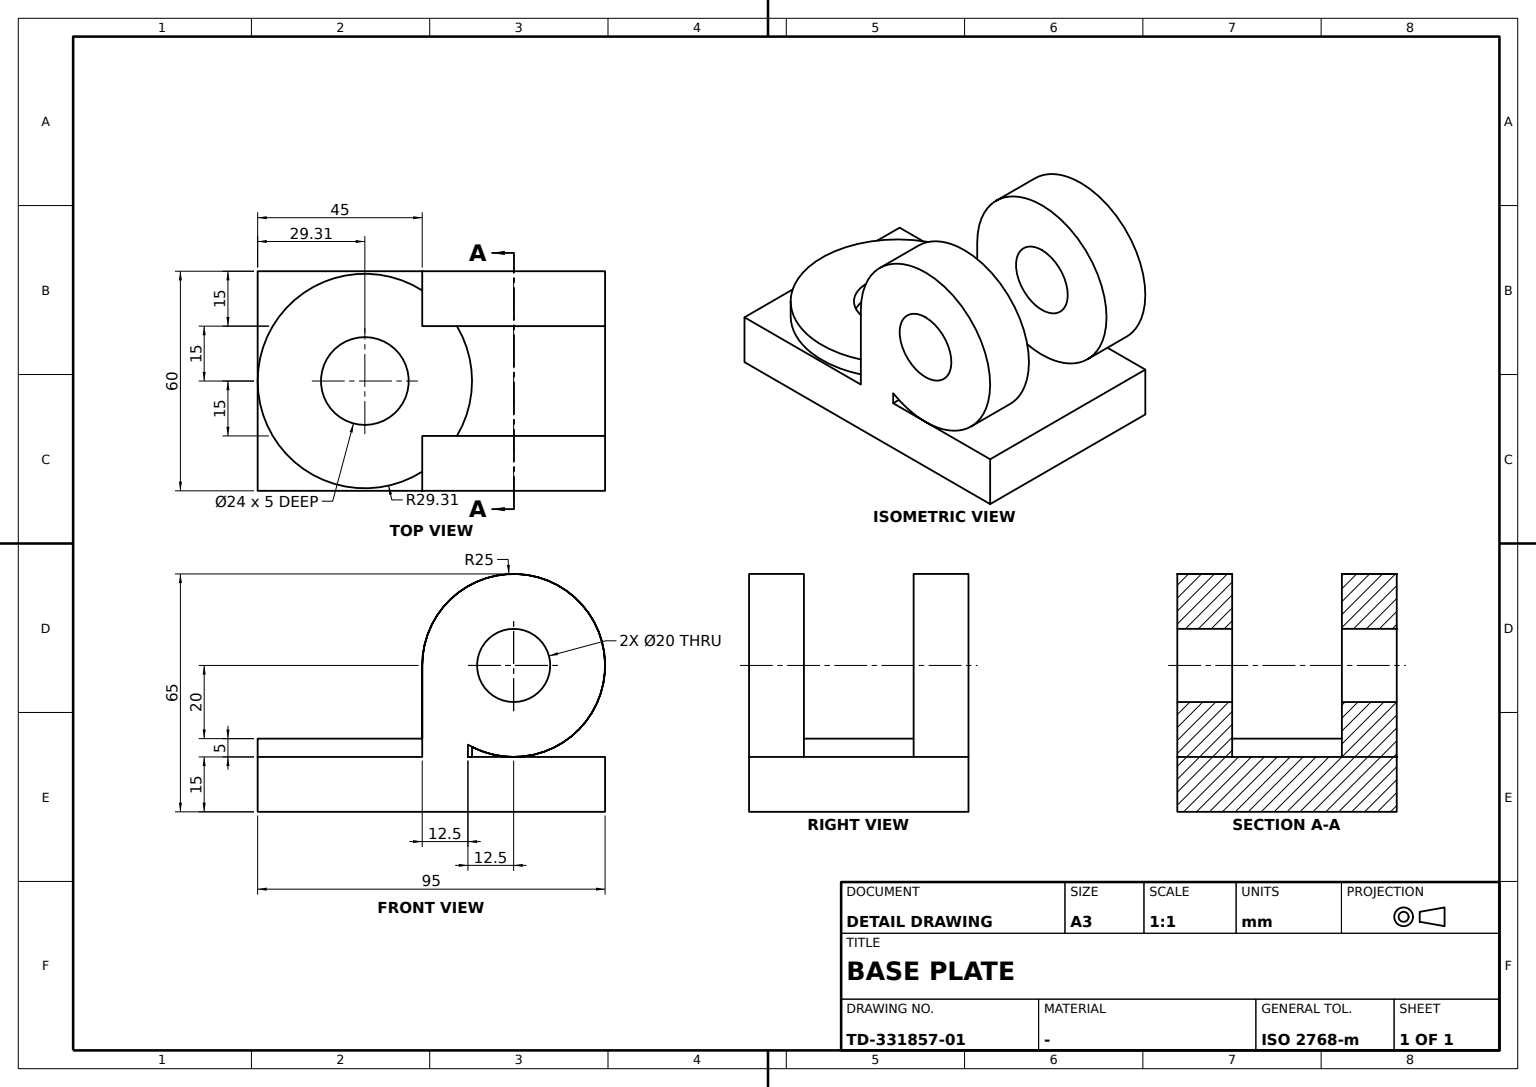
ISO-10303-21;
HEADER;
FILE_DESCRIPTION((''),'2;1');
FILE_NAME('','',(''),(''),'','','');
FILE_SCHEMA(('AUTOMOTIVE_DESIGN'));
ENDSEC;
DATA;
#1=APPLICATION_CONTEXT('');
#2=PRODUCT_CONTEXT('',#1,'mechanical');
#3=PRODUCT('','','',(#2));
#4=PRODUCT_DEFINITION_FORMATION('','',#3);
#5=PRODUCT_DEFINITION_CONTEXT('',#1,'design');
#6=PRODUCT_DEFINITION('','',#4,#5);
#7=PRODUCT_DEFINITION_SHAPE('','',#6);
#8=(LENGTH_UNIT()NAMED_UNIT(*)SI_UNIT(.MILLI.,.METRE.));
#9=(NAMED_UNIT(*)PLANE_ANGLE_UNIT()SI_UNIT($,.RADIAN.));
#10=(NAMED_UNIT(*)SI_UNIT($,.STERADIAN.)SOLID_ANGLE_UNIT());
#11=UNCERTAINTY_MEASURE_WITH_UNIT(LENGTH_MEASURE(0.005),#8,'distance_accuracy_value','');
#12=(GEOMETRIC_REPRESENTATION_CONTEXT(3)GLOBAL_UNCERTAINTY_ASSIGNED_CONTEXT((#11))GLOBAL_UNIT_ASSIGNED_CONTEXT((#8,#9,#10))REPRESENTATION_CONTEXT('',''));
#13=CARTESIAN_POINT('',(-15.,22.5,50.));
#14=VERTEX_POINT('',#13);
#15=CARTESIAN_POINT('',(-15.,22.5,40.));
#16=DIRECTION('',(-1.,0.,0.));
#17=DIRECTION('',(0.,0.,1.));
#18=AXIS2_PLACEMENT_3D('',#15,#16,#17);
#19=CIRCLE('',#18,10.);
#20=EDGE_CURVE('',#14,#14,#19,.T.);
#21=ORIENTED_EDGE('',*,*,#20,.T.);
#22=EDGE_LOOP('',(#21));
#23=FACE_BOUND('',#22,.T.);
#24=CARTESIAN_POINT('',(-15.,-2.5,40.));
#25=VERTEX_POINT('',#24);
#26=CARTESIAN_POINT('',(-15.,10.,18.349365));
#27=VERTEX_POINT('',#26);
#28=CIRCLE('',#18,25.);
#29=EDGE_CURVE('',#25,#27,#28,.T.);
#30=ORIENTED_EDGE('',*,*,#29,.F.);
#31=CARTESIAN_POINT('',(-15.,-2.5,20.));
#32=VERTEX_POINT('',#31);
#33=DIRECTION('',(0.,0.,-1.));
#34=VECTOR('',#33,1000.);
#35=LINE('',#24,#34);
#36=EDGE_CURVE('',#25,#32,#35,.T.);
#37=ORIENTED_EDGE('',*,*,#36,.T.);
#38=CARTESIAN_POINT('',(-15.,6.991539,20.));
#39=VERTEX_POINT('',#38);
#40=CARTESIAN_POINT('',(-15.,0.,20.));
#41=DIRECTION('',(0.,-1.,0.));
#42=VECTOR('',#41,1000.);
#43=LINE('',#40,#42);
#44=EDGE_CURVE('',#39,#32,#43,.T.);
#45=ORIENTED_EDGE('',*,*,#44,.F.);
#46=CARTESIAN_POINT('',(-15.,6.991539,15.));
#47=VERTEX_POINT('',#46);
#48=VECTOR('',#17,1000.);
#49=LINE('',#46,#48);
#50=EDGE_CURVE('',#47,#39,#49,.T.);
#51=ORIENTED_EDGE('',*,*,#50,.F.);
#52=CARTESIAN_POINT('',(-15.,10.,15.));
#53=VERTEX_POINT('',#52);
#54=CARTESIAN_POINT('',(-15.,0.,15.));
#55=DIRECTION('',(0.,1.,0.));
#56=VECTOR('',#55,1000.);
#57=LINE('',#54,#56);
#58=EDGE_CURVE('',#47,#53,#57,.T.);
#59=ORIENTED_EDGE('',*,*,#58,.T.);
#60=LINE('',#52,#48);
#61=EDGE_CURVE('',#53,#27,#60,.T.);
#62=ORIENTED_EDGE('',*,*,#61,.T.);
#63=EDGE_LOOP('',(#30,#37,#45,#51,#59,#62));
#64=FACE_BOUND('',#63,.T.);
#65=CARTESIAN_POINT('',(-15.,0.,0.));
#66=AXIS2_PLACEMENT_3D('',#65,#16,#41);
#67=PLANE('',#66);
#68=ADVANCED_FACE('',(#23,#64),#67,.F.);
#69=CARTESIAN_POINT('',(-24.757381,-2.5,20.));
#70=VERTEX_POINT('',#69);
#71=CARTESIAN_POINT('',(24.757381,-2.5,20.));
#72=VERTEX_POINT('',#71);
#73=CARTESIAN_POINT('',(0.,-18.18969,20.));
#74=DIRECTION('',(1.,0.,0.));
#75=AXIS2_PLACEMENT_3D('',#73,#17,#74);
#76=CIRCLE('',#75,29.31031);
#77=EDGE_CURVE('',#70,#72,#76,.T.);
#78=ORIENTED_EDGE('',*,*,#77,.F.);
#79=CARTESIAN_POINT('',(-24.757381,-2.5,15.));
#80=VERTEX_POINT('',#79);
#81=LINE('',#79,#48);
#82=EDGE_CURVE('',#80,#70,#81,.T.);
#83=ORIENTED_EDGE('',*,*,#82,.F.);
#84=CARTESIAN_POINT('',(0.,-47.5,15.));
#85=VERTEX_POINT('',#84);
#86=CARTESIAN_POINT('',(0.,-18.18969,15.));
#87=AXIS2_PLACEMENT_3D('',#86,#17,#74);
#88=CIRCLE('',#87,29.31031);
#89=EDGE_CURVE('',#80,#85,#88,.T.);
#90=ORIENTED_EDGE('',*,*,#89,.T.);
#91=CARTESIAN_POINT('',(24.757381,-2.5,15.));
#92=VERTEX_POINT('',#91);
#93=EDGE_CURVE('',#85,#92,#88,.T.);
#94=ORIENTED_EDGE('',*,*,#93,.T.);
#95=LINE('',#91,#48);
#96=EDGE_CURVE('',#92,#72,#95,.T.);
#97=ORIENTED_EDGE('',*,*,#96,.T.);
#98=EDGE_LOOP('',(#78,#83,#90,#94,#97));
#99=FACE_BOUND('',#98,.T.);
#100=CARTESIAN_POINT('',(0.,-18.18969,17.5));
#101=AXIS2_PLACEMENT_3D('',#100,#17,#74);
#102=CYLINDRICAL_SURFACE('',#101,29.31031);
#103=ADVANCED_FACE('',(#99),#102,.T.);
#104=CARTESIAN_POINT('',(-30.,-2.5,40.));
#105=VERTEX_POINT('',#104);
#106=CARTESIAN_POINT('',(-30.,10.,18.349365));
#107=VERTEX_POINT('',#106);
#108=CARTESIAN_POINT('',(-30.,22.5,40.));
#109=AXIS2_PLACEMENT_3D('',#108,#16,#17);
#110=CIRCLE('',#109,25.);
#111=EDGE_CURVE('',#105,#107,#110,.T.);
#112=ORIENTED_EDGE('',*,*,#111,.F.);
#113=CARTESIAN_POINT('',(-22.5,-2.5,40.));
#114=VECTOR('',#16,1000.);
#115=LINE('',#113,#114);
#116=EDGE_CURVE('',#105,#25,#115,.F.);
#117=ORIENTED_EDGE('',*,*,#116,.T.);
#118=ORIENTED_EDGE('',*,*,#29,.T.);
#119=LINE('',#106,#114);
#120=EDGE_CURVE('',#107,#27,#119,.F.);
#121=ORIENTED_EDGE('',*,*,#120,.F.);
#122=EDGE_LOOP('',(#112,#117,#118,#121));
#123=FACE_BOUND('',#122,.T.);
#124=CARTESIAN_POINT('',(-22.5,22.5,40.));
#125=AXIS2_PLACEMENT_3D('',#124,#16,#41);
#126=CYLINDRICAL_SURFACE('',#125,25.);
#127=ADVANCED_FACE('',(#123),#126,.T.);
#128=CARTESIAN_POINT('',(12.,-18.18969,20.));
#129=VERTEX_POINT('',#128);
#130=CIRCLE('',#75,12.);
#131=EDGE_CURVE('',#129,#129,#130,.T.);
#132=ORIENTED_EDGE('',*,*,#131,.T.);
#133=EDGE_LOOP('',(#132));
#134=FACE_BOUND('',#133,.T.);
#135=CARTESIAN_POINT('',(12.,-18.18969,15.));
#136=VERTEX_POINT('',#135);
#137=CIRCLE('',#87,12.);
#138=EDGE_CURVE('',#136,#136,#137,.T.);
#139=ORIENTED_EDGE('',*,*,#138,.F.);
#140=EDGE_LOOP('',(#139));
#141=FACE_BOUND('',#140,.T.);
#142=CYLINDRICAL_SURFACE('',#101,12.);
#143=ADVANCED_FACE('',(#134,#141),#142,.F.);
#144=CARTESIAN_POINT('',(30.,22.5,15.));
#145=VERTEX_POINT('',#144);
#146=CARTESIAN_POINT('',(30.,10.,18.349365));
#147=VERTEX_POINT('',#146);
#148=CARTESIAN_POINT('',(30.,22.5,40.));
#149=AXIS2_PLACEMENT_3D('',#148,#16,#17);
#150=CIRCLE('',#149,25.);
#151=EDGE_CURVE('',#145,#147,#150,.T.);
#152=ORIENTED_EDGE('',*,*,#151,.T.);
#153=CARTESIAN_POINT('',(15.,10.,18.349365));
#154=VERTEX_POINT('',#153);
#155=LINE('',#153,#114);
#156=EDGE_CURVE('',#154,#147,#155,.F.);
#157=ORIENTED_EDGE('',*,*,#156,.F.);
#158=CARTESIAN_POINT('',(15.,-2.5,40.));
#159=VERTEX_POINT('',#158);
#160=CARTESIAN_POINT('',(15.,22.5,40.));
#161=AXIS2_PLACEMENT_3D('',#160,#16,#17);
#162=CIRCLE('',#161,25.);
#163=EDGE_CURVE('',#159,#154,#162,.T.);
#164=ORIENTED_EDGE('',*,*,#163,.F.);
#165=CARTESIAN_POINT('',(30.,-2.5,40.));
#166=VERTEX_POINT('',#165);
#167=EDGE_CURVE('',#159,#166,#115,.F.);
#168=ORIENTED_EDGE('',*,*,#167,.T.);
#169=EDGE_CURVE('',#166,#145,#150,.T.);
#170=ORIENTED_EDGE('',*,*,#169,.T.);
#171=EDGE_LOOP('',(#152,#157,#164,#168,#170));
#172=FACE_BOUND('',#171,.T.);
#173=ADVANCED_FACE('',(#172),#126,.T.);
#174=ORIENTED_EDGE('',*,*,#50,.T.);
#175=CARTESIAN_POINT('',(15.,6.991539,20.));
#176=VERTEX_POINT('',#175);
#177=EDGE_CURVE('',#176,#39,#76,.T.);
#178=ORIENTED_EDGE('',*,*,#177,.F.);
#179=CARTESIAN_POINT('',(15.,6.991539,15.));
#180=VERTEX_POINT('',#179);
#181=LINE('',#179,#48);
#182=EDGE_CURVE('',#180,#176,#181,.T.);
#183=ORIENTED_EDGE('',*,*,#182,.F.);
#184=EDGE_CURVE('',#180,#47,#88,.T.);
#185=ORIENTED_EDGE('',*,*,#184,.T.);
#186=EDGE_LOOP('',(#174,#178,#183,#185));
#187=FACE_BOUND('',#186,.T.);
#188=ADVANCED_FACE('',(#187),#102,.T.);
#189=ORIENTED_EDGE('',*,*,#138,.T.);
#190=EDGE_LOOP('',(#189));
#191=FACE_BOUND('',#190,.T.);
#192=CARTESIAN_POINT('',(0.,0.,15.));
#193=AXIS2_PLACEMENT_3D('',#192,#17,#74);
#194=PLANE('',#193);
#195=ADVANCED_FACE('',(#191),#194,.T.);
#196=CARTESIAN_POINT('',(-30.,22.5,50.));
#197=VERTEX_POINT('',#196);
#198=CIRCLE('',#109,10.);
#199=EDGE_CURVE('',#197,#197,#198,.T.);
#200=ORIENTED_EDGE('',*,*,#199,.T.);
#201=EDGE_LOOP('',(#200));
#202=FACE_BOUND('',#201,.T.);
#203=ORIENTED_EDGE('',*,*,#20,.F.);
#204=EDGE_LOOP('',(#203));
#205=FACE_BOUND('',#204,.T.);
#206=CYLINDRICAL_SURFACE('',#125,10.);
#207=ADVANCED_FACE('',(#202,#205),#206,.F.);
#208=CARTESIAN_POINT('',(-30.,47.5,0.));
#209=VERTEX_POINT('',#208);
#210=CARTESIAN_POINT('',(30.,47.5,0.));
#211=VERTEX_POINT('',#210);
#212=CARTESIAN_POINT('',(0.,47.5,0.));
#213=VECTOR('',#74,1000.);
#214=LINE('',#212,#213);
#215=EDGE_CURVE('',#209,#211,#214,.T.);
#216=ORIENTED_EDGE('',*,*,#215,.F.);
#217=CARTESIAN_POINT('',(-30.,47.5,15.));
#218=VERTEX_POINT('',#217);
#219=LINE('',#208,#48);
#220=EDGE_CURVE('',#209,#218,#219,.T.);
#221=ORIENTED_EDGE('',*,*,#220,.T.);
#222=CARTESIAN_POINT('',(30.,47.5,15.));
#223=VERTEX_POINT('',#222);
#224=CARTESIAN_POINT('',(0.,47.5,15.));
#225=LINE('',#224,#213);
#226=EDGE_CURVE('',#218,#223,#225,.T.);
#227=ORIENTED_EDGE('',*,*,#226,.T.);
#228=LINE('',#210,#48);
#229=EDGE_CURVE('',#211,#223,#228,.T.);
#230=ORIENTED_EDGE('',*,*,#229,.F.);
#231=EDGE_LOOP('',(#216,#221,#227,#230));
#232=FACE_BOUND('',#231,.T.);
#233=AXIS2_PLACEMENT_3D('',#208,#41,#74);
#234=PLANE('',#233);
#235=ADVANCED_FACE('',(#232),#234,.F.);
#236=CARTESIAN_POINT('',(-30.,-2.5,15.));
#237=VERTEX_POINT('',#236);
#238=LINE('',#104,#34);
#239=EDGE_CURVE('',#105,#237,#238,.T.);
#240=ORIENTED_EDGE('',*,*,#239,.F.);
#241=ORIENTED_EDGE('',*,*,#111,.T.);
#242=CARTESIAN_POINT('',(-30.,10.,15.));
#243=VERTEX_POINT('',#242);
#244=LINE('',#242,#48);
#245=EDGE_CURVE('',#243,#107,#244,.T.);
#246=ORIENTED_EDGE('',*,*,#245,.F.);
#247=CARTESIAN_POINT('',(-30.,0.,15.));
#248=LINE('',#247,#42);
#249=EDGE_CURVE('',#218,#243,#248,.T.);
#250=ORIENTED_EDGE('',*,*,#249,.F.);
#251=ORIENTED_EDGE('',*,*,#220,.F.);
#252=CARTESIAN_POINT('',(-30.,-47.5,0.));
#253=VERTEX_POINT('',#252);
#254=CARTESIAN_POINT('',(-30.,0.,0.));
#255=LINE('',#254,#42);
#256=EDGE_CURVE('',#209,#253,#255,.T.);
#257=ORIENTED_EDGE('',*,*,#256,.T.);
#258=CARTESIAN_POINT('',(-30.,-47.5,15.));
#259=VERTEX_POINT('',#258);
#260=LINE('',#252,#48);
#261=EDGE_CURVE('',#253,#259,#260,.T.);
#262=ORIENTED_EDGE('',*,*,#261,.T.);
#263=EDGE_CURVE('',#237,#259,#248,.T.);
#264=ORIENTED_EDGE('',*,*,#263,.F.);
#265=EDGE_LOOP('',(#240,#241,#246,#250,#251,#257,#262,#264));
#266=FACE_BOUND('',#265,.T.);
#267=ORIENTED_EDGE('',*,*,#199,.F.);
#268=EDGE_LOOP('',(#267));
#269=FACE_BOUND('',#268,.T.);
#270=AXIS2_PLACEMENT_3D('',#208,#16,#41);
#271=PLANE('',#270);
#272=ADVANCED_FACE('',(#266,#269),#271,.T.);
#273=CARTESIAN_POINT('',(15.,-2.5,20.));
#274=VERTEX_POINT('',#273);
#275=CARTESIAN_POINT('',(0.,-2.5,20.));
#276=LINE('',#275,#213);
#277=EDGE_CURVE('',#274,#72,#276,.T.);
#278=ORIENTED_EDGE('',*,*,#277,.T.);
#279=ORIENTED_EDGE('',*,*,#96,.F.);
#280=CARTESIAN_POINT('',(30.,-2.5,15.));
#281=VERTEX_POINT('',#280);
#282=CARTESIAN_POINT('',(0.,-2.5,15.));
#283=LINE('',#282,#213);
#284=EDGE_CURVE('',#92,#281,#283,.T.);
#285=ORIENTED_EDGE('',*,*,#284,.T.);
#286=LINE('',#165,#34);
#287=EDGE_CURVE('',#166,#281,#286,.T.);
#288=ORIENTED_EDGE('',*,*,#287,.F.);
#289=ORIENTED_EDGE('',*,*,#167,.F.);
#290=LINE('',#158,#34);
#291=EDGE_CURVE('',#159,#274,#290,.T.);
#292=ORIENTED_EDGE('',*,*,#291,.T.);
#293=EDGE_LOOP('',(#278,#279,#285,#288,#289,#292));
#294=FACE_BOUND('',#293,.T.);
#295=AXIS2_PLACEMENT_3D('',#104,#41,#33);
#296=PLANE('',#295);
#297=ADVANCED_FACE('',(#294),#296,.T.);
#298=ORIENTED_EDGE('',*,*,#61,.F.);
#299=LINE('',#242,#213);
#300=EDGE_CURVE('',#243,#53,#299,.T.);
#301=ORIENTED_EDGE('',*,*,#300,.F.);
#302=ORIENTED_EDGE('',*,*,#245,.T.);
#303=ORIENTED_EDGE('',*,*,#120,.T.);
#304=EDGE_LOOP('',(#298,#301,#302,#303));
#305=FACE_BOUND('',#304,.T.);
#306=AXIS2_PLACEMENT_3D('',#242,#55,#17);
#307=PLANE('',#306);
#308=ADVANCED_FACE('',(#305),#307,.T.);
#309=ORIENTED_EDGE('',*,*,#215,.T.);
#310=CARTESIAN_POINT('',(30.,-47.5,0.));
#311=VERTEX_POINT('',#310);
#312=LINE('',#210,#56);
#313=EDGE_CURVE('',#311,#211,#312,.T.);
#314=ORIENTED_EDGE('',*,*,#313,.F.);
#315=CARTESIAN_POINT('',(0.,-47.5,0.));
#316=LINE('',#315,#114);
#317=EDGE_CURVE('',#311,#253,#316,.T.);
#318=ORIENTED_EDGE('',*,*,#317,.T.);
#319=ORIENTED_EDGE('',*,*,#256,.F.);
#320=EDGE_LOOP('',(#309,#314,#318,#319));
#321=FACE_BOUND('',#320,.T.);
#322=CARTESIAN_POINT('',(0.,0.,0.));
#323=AXIS2_PLACEMENT_3D('',#322,#17,#74);
#324=PLANE('',#323);
#325=ADVANCED_FACE('',(#321),#324,.F.);
#326=ORIENTED_EDGE('',*,*,#82,.T.);
#327=EDGE_CURVE('',#70,#32,#276,.T.);
#328=ORIENTED_EDGE('',*,*,#327,.T.);
#329=ORIENTED_EDGE('',*,*,#36,.F.);
#330=ORIENTED_EDGE('',*,*,#116,.F.);
#331=ORIENTED_EDGE('',*,*,#239,.T.);
#332=EDGE_CURVE('',#237,#80,#283,.T.);
#333=ORIENTED_EDGE('',*,*,#332,.T.);
#334=EDGE_LOOP('',(#326,#328,#329,#330,#331,#333));
#335=FACE_BOUND('',#334,.T.);
#336=ADVANCED_FACE('',(#335),#296,.T.);
#337=ORIENTED_EDGE('',*,*,#184,.F.);
#338=CARTESIAN_POINT('',(15.,10.,15.));
#339=VERTEX_POINT('',#338);
#340=CARTESIAN_POINT('',(15.,0.,15.));
#341=LINE('',#340,#56);
#342=EDGE_CURVE('',#180,#339,#341,.T.);
#343=ORIENTED_EDGE('',*,*,#342,.T.);
#344=CARTESIAN_POINT('',(30.,10.,15.));
#345=VERTEX_POINT('',#344);
#346=EDGE_CURVE('',#339,#345,#299,.T.);
#347=ORIENTED_EDGE('',*,*,#346,.T.);
#348=LINE('',#222,#56);
#349=EDGE_CURVE('',#345,#145,#348,.T.);
#350=ORIENTED_EDGE('',*,*,#349,.T.);
#351=EDGE_CURVE('',#145,#223,#348,.T.);
#352=ORIENTED_EDGE('',*,*,#351,.T.);
#353=ORIENTED_EDGE('',*,*,#226,.F.);
#354=ORIENTED_EDGE('',*,*,#249,.T.);
#355=ORIENTED_EDGE('',*,*,#300,.T.);
#356=ORIENTED_EDGE('',*,*,#58,.F.);
#357=EDGE_LOOP('',(#337,#343,#347,#350,#352,#353,#354,#355,#356));
#358=FACE_BOUND('',#357,.T.);
#359=ADVANCED_FACE('',(#358),#194,.T.);
#360=CARTESIAN_POINT('',(30.,-47.5,15.));
#361=VERTEX_POINT('',#360);
#362=LINE('',#310,#48);
#363=EDGE_CURVE('',#311,#361,#362,.T.);
#364=ORIENTED_EDGE('',*,*,#363,.T.);
#365=LINE('',#84,#114);
#366=EDGE_CURVE('',#361,#85,#365,.T.);
#367=ORIENTED_EDGE('',*,*,#366,.T.);
#368=EDGE_CURVE('',#85,#259,#365,.T.);
#369=ORIENTED_EDGE('',*,*,#368,.T.);
#370=ORIENTED_EDGE('',*,*,#261,.F.);
#371=ORIENTED_EDGE('',*,*,#317,.F.);
#372=EDGE_LOOP('',(#364,#367,#369,#370,#371));
#373=FACE_BOUND('',#372,.T.);
#374=AXIS2_PLACEMENT_3D('',#310,#55,#16);
#375=PLANE('',#374);
#376=ADVANCED_FACE('',(#373),#375,.F.);
#377=CARTESIAN_POINT('',(15.,22.5,50.));
#378=VERTEX_POINT('',#377);
#379=CIRCLE('',#161,10.);
#380=EDGE_CURVE('',#378,#378,#379,.T.);
#381=ORIENTED_EDGE('',*,*,#380,.T.);
#382=EDGE_LOOP('',(#381));
#383=FACE_BOUND('',#382,.T.);
#384=CARTESIAN_POINT('',(30.,22.5,50.));
#385=VERTEX_POINT('',#384);
#386=CIRCLE('',#149,10.);
#387=EDGE_CURVE('',#385,#385,#386,.T.);
#388=ORIENTED_EDGE('',*,*,#387,.F.);
#389=EDGE_LOOP('',(#388));
#390=FACE_BOUND('',#389,.T.);
#391=ADVANCED_FACE('',(#383,#390),#206,.F.);
#392=ORIENTED_EDGE('',*,*,#380,.F.);
#393=EDGE_LOOP('',(#392));
#394=FACE_BOUND('',#393,.T.);
#395=CARTESIAN_POINT('',(15.,0.,20.));
#396=LINE('',#395,#42);
#397=EDGE_CURVE('',#176,#274,#396,.T.);
#398=ORIENTED_EDGE('',*,*,#397,.T.);
#399=ORIENTED_EDGE('',*,*,#291,.F.);
#400=ORIENTED_EDGE('',*,*,#163,.T.);
#401=LINE('',#338,#48);
#402=EDGE_CURVE('',#339,#154,#401,.T.);
#403=ORIENTED_EDGE('',*,*,#402,.F.);
#404=ORIENTED_EDGE('',*,*,#342,.F.);
#405=ORIENTED_EDGE('',*,*,#182,.T.);
#406=EDGE_LOOP('',(#398,#399,#400,#403,#404,#405));
#407=FACE_BOUND('',#406,.T.);
#408=CARTESIAN_POINT('',(15.,0.,0.));
#409=AXIS2_PLACEMENT_3D('',#408,#16,#41);
#410=PLANE('',#409);
#411=ADVANCED_FACE('',(#394,#407),#410,.T.);
#412=ORIENTED_EDGE('',*,*,#131,.F.);
#413=EDGE_LOOP('',(#412));
#414=FACE_BOUND('',#413,.T.);
#415=ORIENTED_EDGE('',*,*,#397,.F.);
#416=ORIENTED_EDGE('',*,*,#177,.T.);
#417=ORIENTED_EDGE('',*,*,#44,.T.);
#418=ORIENTED_EDGE('',*,*,#327,.F.);
#419=ORIENTED_EDGE('',*,*,#77,.T.);
#420=ORIENTED_EDGE('',*,*,#277,.F.);
#421=EDGE_LOOP('',(#415,#416,#417,#418,#419,#420));
#422=FACE_BOUND('',#421,.T.);
#423=CARTESIAN_POINT('',(0.,0.,20.));
#424=AXIS2_PLACEMENT_3D('',#423,#17,#74);
#425=PLANE('',#424);
#426=ADVANCED_FACE('',(#414,#422),#425,.T.);
#427=ORIENTED_EDGE('',*,*,#387,.T.);
#428=EDGE_LOOP('',(#427));
#429=FACE_BOUND('',#428,.T.);
#430=ORIENTED_EDGE('',*,*,#313,.T.);
#431=ORIENTED_EDGE('',*,*,#229,.T.);
#432=ORIENTED_EDGE('',*,*,#351,.F.);
#433=ORIENTED_EDGE('',*,*,#169,.F.);
#434=ORIENTED_EDGE('',*,*,#287,.T.);
#435=EDGE_CURVE('',#361,#281,#348,.T.);
#436=ORIENTED_EDGE('',*,*,#435,.F.);
#437=ORIENTED_EDGE('',*,*,#363,.F.);
#438=EDGE_LOOP('',(#430,#431,#432,#433,#434,#436,#437));
#439=FACE_BOUND('',#438,.T.);
#440=LINE('',#344,#48);
#441=EDGE_CURVE('',#345,#147,#440,.T.);
#442=ORIENTED_EDGE('',*,*,#441,.T.);
#443=ORIENTED_EDGE('',*,*,#151,.F.);
#444=ORIENTED_EDGE('',*,*,#349,.F.);
#445=EDGE_LOOP('',(#442,#443,#444));
#446=FACE_BOUND('',#445,.T.);
#447=AXIS2_PLACEMENT_3D('',#210,#16,#41);
#448=PLANE('',#447);
#449=ADVANCED_FACE('',(#429,#439,#446),#448,.F.);
#450=ORIENTED_EDGE('',*,*,#263,.T.);
#451=ORIENTED_EDGE('',*,*,#368,.F.);
#452=ORIENTED_EDGE('',*,*,#89,.F.);
#453=ORIENTED_EDGE('',*,*,#332,.F.);
#454=EDGE_LOOP('',(#450,#451,#452,#453));
#455=FACE_BOUND('',#454,.T.);
#456=ADVANCED_FACE('',(#455),#194,.T.);
#457=ORIENTED_EDGE('',*,*,#441,.F.);
#458=ORIENTED_EDGE('',*,*,#346,.F.);
#459=ORIENTED_EDGE('',*,*,#402,.T.);
#460=ORIENTED_EDGE('',*,*,#156,.T.);
#461=EDGE_LOOP('',(#457,#458,#459,#460));
#462=FACE_BOUND('',#461,.T.);
#463=ADVANCED_FACE('',(#462),#307,.T.);
#464=ORIENTED_EDGE('',*,*,#366,.F.);
#465=ORIENTED_EDGE('',*,*,#435,.T.);
#466=ORIENTED_EDGE('',*,*,#284,.F.);
#467=ORIENTED_EDGE('',*,*,#93,.F.);
#468=EDGE_LOOP('',(#464,#465,#466,#467));
#469=FACE_BOUND('',#468,.T.);
#470=ADVANCED_FACE('',(#469),#194,.T.);
#471=CLOSED_SHELL('',(#68,#103,#127,#143,#173,#188,#195,#207,#235,#272,#297,#308,#325,#336,#359,#376,#391,#411,#426,#449,#456,#463,#470));
#472=MANIFOLD_SOLID_BREP('',#471);
#473=ADVANCED_BREP_SHAPE_REPRESENTATION('',(#472),#12);
#474=SHAPE_DEFINITION_REPRESENTATION(#7,#473);
ENDSEC;
END-ISO-10303-21;
